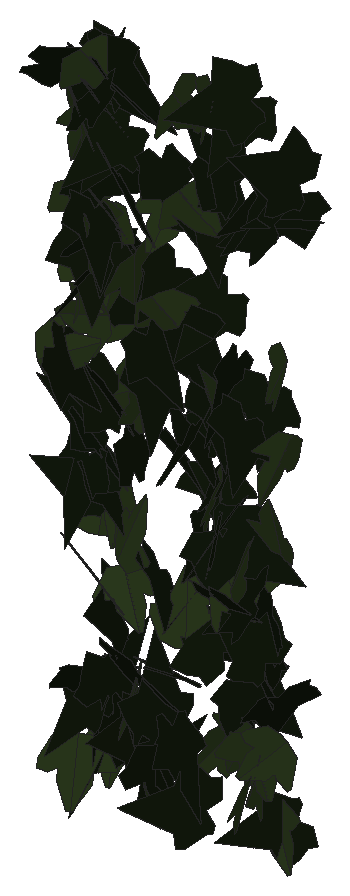
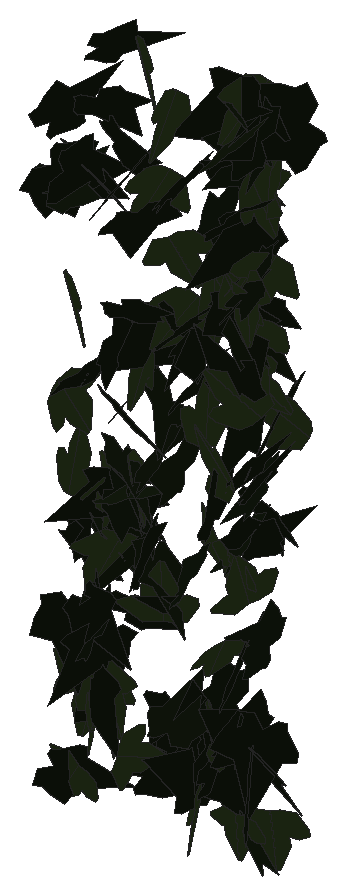
# SketchUp Ruby script. Lengths in inches.
U = 1.inch
M = Sketchup.active_model
def pt(a) = Geom::Point3d.new(a.map { |v| v * U })
def face(e, loops, mat)
  f = e.add_face(loops[0].map { |a| pt(a) })
  loops[1..].each { |l| e.add_face(l.map { |a| pt(a) }).erase! }
  f.material = f.back_material = mat if mat
  f
end
# faces: each face lists its corners as indices into pts; further lists are holes
def faces(e, pts, list, mat = nil) = list.each { |f| face(e, (f[0].is_a?(Array) ? f : [f]).map { |l| l.map { |i| pts[i] } }, mat) }
# xy, xz, yz: faces in a plane at the given z, y or x. An outline is a flat list of corners, or four numbers for a rectangle; further outlines are holes
def ring(l) = l.size == 4 ? [[l[0], l[1]], [l[2], l[1]], [l[2], l[3]], [l[0], l[3]]] : l.each_slice(2).to_a
def flat(e, list, mat, &to3) = list.each { |f| face(e, (f[0].is_a?(Array) ? f : [f]).map { |l| ring(l).map { |u, v| to3.(u, v) } }, mat) }
def xy(e, z, list, mat = nil) = flat(e, list, mat) { |x, y| [x, y, z] }
def xz(e, y, list, mat = nil) = flat(e, list, mat) { |x, z| [x, y, z] }
def yz(e, x, list, mat = nil) = flat(e, list, mat) { |y, z| [x, y, z] }
def lines(e, pts, list) = list.each { |a, b| e.add_line(pt(pts[a]), pt(pts[b])) }
# prism: a flat outline (further loops are holes) pulled along v
def prism(e, loops, v, mat = nil)
  f = face(e, loops, mat); d = Geom::Vector3d.new(v.map { |x| x * U })
  f.pushpull(f.normal.samedirection?(d) ? d.length : -d.length)
end
def box(e, o, s, mat = nil) = prism(e, [[o, [o[0] + s[0], o[1], o[2]], [o[0] + s[0], o[1] + s[1], o[2]], [o[0], o[1] + s[1], o[2]]]], [0, 0, s[2]], mat)
def at(x, y, z, deg = 0) = Geom::Transformation.translation(pt([x, y, z])) * Geom::Transformation.rotation(ORIGIN, Z_AXIS, deg.degrees)
def axes(o, x, y, z) = Geom::Transformation.new([*x, 0, *y, 0, *z, 0, *pt(o).to_a, 1])
def part(name) = M.definitions.add(name)
# library, detail: a bought-in or finely detailed component or shape, given as its bounding box
def library(name, o, s) = part(name).tap { |d| box(d.entities, o, s) }
def detail(e, o, s) = box(e.add_group.entities, o, s)
def put(e, d, t, mat = nil) = e.add_instance(d, t).tap { |i| i.material = mat if mat }
def group(e, t, mat = nil) = e.add_group.tap { |g| g.transformation = t; g.material = mat if mat }.entities
root = M.entities
M.materials.add("efeu1").color = [18, 25, 13]
M.materials.add("efeu2").color = [43, 57, 29]
c1 = part("ivyleaf_10")
p = [[0,0.5,-0.03],[-0.0625,2.02,-0.43],[-0.19,2.01,-0.46],[-0.54,1.05,-0.29],[-0.52,0.625,-0.18],[-0.83,0.76,-0.28],
  [-1.16,0.64,-0.33],[-1.15,0.33,-0.24],[-0.77,-0.39,0.02],[-0.3,-0.51,0.16],[0.04,-0.48,0.23],[-0.02,2.01,-0.4375],
  [-0.06,2.01,-0.43],[0.04,-0.49,0.23],[0.67,-0.49,0.14],[1.38,0.36,-0.2],[1.375,0.51,-0.24],[0.81,0.65,-0.19],
  [0.62,0.59,-0.15],[0.6,1.09,-0.28],[0.5,1.23,-0.31]]
faces(c1.entities,p,[[0,1,2,3,4,5,6,7,8,9,10],[11,12,0,13,14,15,16,17,18,19,20]],"efeu2")
c2 = part("ivyleaf_9")
p = [[1.54,2.16,1.25],[1.36,2.04,1.19],[-0.21,0.99,0.68],[-0.71,1.11,0.82],[-0.85,0.86,0.67],[-0.8,0.17,0.21],
  [-0.9,-0.01,0.1],[-0.67,-0.16,-0.02],[-0.08,-0.08,-0.05],[-0.03,-0.6,-0.4],[0.65,-0.88,-0.66],[0.83,-0.6,-0.49],
  [1.29,-0.42,-0.43],[1.8125,-0.07,-0.26],[1.21,0.44,0.15]]
faces(c2.entities,p,[[0,1,2,3,4,5,6,7,8,9,10,11,12,13,14]],"efeu1")
put(root,c1,axes([584.58,125.34,243.96],[1.0955,0.54995,-0.00416],[-0.00399,-0.00134,-1.22579],[-0.54995,1.0955,0.00059]))
put(root,c1,axes([583.95,124.68,261.51],[0.54254,-0.06384,-1.07288],[1.0655,-0.1256,0.54628],[-0.14089,-1.19567,-0.0001]))
put(root,c2,axes([584.14,123.93,274.76],[1.02793,0.37138,0.65667],[0.58931,0.29764,-1.09083],[-0.47101,1.18291,0.06831]))
put(root,c1,axes([584.64,125.48,268.77],[-0.86196,-0.52468,-0.46844],[0.52456,0.01409,-0.98099],[0.46858,-0.98093,0.23648]))
put(root,c1,axes([585.66,125.26,263.58],[0.41861,-0.1033,-1.10017],[-1.02006,0.41622,-0.42721],[0.42487,1.10107,0.05828]))
put(root,c1,axes([585.06,125.76,272.39],[-0.07314,-1.11185,0.34435],[-0.01366,-0.34419,-1.11422],[1.16387,-0.07391,0.00856]))
put(root,c2,axes([585.3,125.53,246.625],[-1.08694,0.11287,-0.22951],[0.22673,-0.03848,-1.09269],[-0.11836,-1.11024,0.01454]))
put(root,c2,axes([584.98,126.36,243.74],[-0.72617,0.2,-0.69404],[0.61757,-0.33844,-0.74369],[-0.37456,-0.94576,0.11936]))
put(root,c2,axes([585.09,125.35,247.72],[0.49911,1.03868,-0.22985],[-0.10203,-0.20597,-1.15237],[-1.0589,0.50943,0.0027]))
put(root,c1,axes([585.41,124.93,271.6],[-0.89919,0.64453,-0.4114],[-0.35391,0.21212,1.10588],[0.6778,0.96582,0.03166]))
put(root,c1,axes([585.42,126.1,267.99],[-1.08113,0.1071,0.42641],[-0.42702,0.01361,-1.08609],[-0.10464,-1.1621,0.02658]))
put(root,c2,axes([584.83,123.89,262.34],[0.77046,-0.53644,-0.92719],[-0.66912,0.65087,-0.93258],[0.8365,1.01472,0.10802]))
put(root,c2,axes([585.3,125.77,258.66],[0.06373,-1.18239,-0.08417],[0.03565,-0.08234,1.1837],[-1.18484,-0.06607,0.03109]))
put(root,c2,axes([584.4,127.07,246],[0.03478,-0.20714,-1.31804],[1.22225,-0.52375,0.11456],[-0.535,-1.21001,0.17604]))
put(root,c2,axes([585.39,126.4,259.47],[0.06632,-1.12656,-0.3189],[0.01473,-0.31859,1.12851],[-1.17074,-0.06783,-0.00387]))
put(root,c2,axes([584.37,125.91,252.13],[0.64336,-0.67956,0.58735],[0.42585,-0.40534,-0.93543],[0.79084,0.77109,0.0259]))
put(root,c2,axes([585.85,125.28,255.84],[-0.21206,0.21732,1.04453],[-0.99984,-0.41209,-0.11725],[0.37228,-0.98295,0.28009]))
put(root,c1,axes([585.23,126.02,254.13],[0.48224,0.98953,-0.45958],[0.1745,0.42605,1.10044],[1.07701,-0.5121,0.02749]))
put(root,c2,axes([584.62,126.13,268.57],[0.92581,-0.63304,0.22891],[0.17491,-0.14967,-1.12128],[0.65004,0.94187,-0.02432]))
put(root,c2,axes([585.81,125.49,265.9375],[-0.62118,0.66692,-0.67679],[0.23689,-0.67436,-0.88194],[-0.92017,-0.62383,0.22984]))
put(root,c1,axes([585.11,126.15,262.66],[-0.5218,-0.69168,0.777],[0.42472,0.65186,0.86551],[-0.94961,0.67162,-0.03984]))
put(root,c2,axes([585.77,125.53,266.82],[0.29725,0.91516,-0.57383],[-0.1381,-0.55808,-0.96158],[-1.07132,0.32586,-0.03526]))
put(root,c1,axes([585.27,126.62,244.25],[0.98544,0.08386,0.16592],[0.1662,0.00359,-0.98894],[-0.0833,0.9993,-0.01037]))
put(root,c1,axes([585.04,125.52,266.05],[1.02884,0.35447,0.46656],[0.44326,0.14572,-1.08817],[-0.3832,1.12024,-0.00608]))
put(root,c2,axes([585.6,126.875,271.09],[-0.49895,-0.93329,0.44428],[-0.03147,-0.47939,-1.04238],[1.03316,-0.46532,0.18281]))
put(root,c2,axes([585.14,125.18,258.84],[0.83061,-0.71632,-0.10791],[-0.06554,0.08919,-1.09655],[0.72143,0.83283,0.02462]))
put(root,c2,axes([585.4375,125.21,270.12],[0.10842,-0.01626,-1.24294],[-0.20746,1.22992,-0.03418],[1.22561,0.20963,0.10417]))
put(root,c2,axes([585.52,125.36,266.95],[-0.75343,-0.65875,-0.64537],[0.51421,0.3917,-1.00013],[0.76553,-0.91144,0.03663]))
put(root,c2,axes([585.6875,124.71,257.44],[-0.97025,-0.20215,-0.69409],[0.69891,0.03471,-0.98709],[0.18483,-1.19245,0.08893]))
put(root,c1,axes([585.7,125.13,266.61],[-0.75059,0.77432,0.53057],[0.37563,-0.3748,1.07837],[0.86022,0.83929,-0.00793]))
put(root,c2,axes([585.34,127.11,274.46],[-0.09012,-1.03828,0.50429],[0.28641,-0.51012,-0.9991],[1.11817,0.04699,0.29655]))
put(root,c2,axes([585.32,126.47,263.51],[-0.38171,0.23002,0.98589],[0.85188,-0.49631,0.44562],[0.54699,0.93347,-0.00601]))
put(root,c2,axes([585.44,125.85,267.45],[0.10794,-1.10129,0.33816],[0.07322,-0.33239,-1.10589],[1.14971,0.12456,0.03869]))
put(root,c2,axes([585.87,126.45,249.92],[-0.21225,-0.19899,1.26782],[-0.17045,-1.26929,-0.22776],[1.27197,-0.2033,0.18104]))
put(root,c2,axes([585.43,125.25,273.52],[1.01366,-0.56525,0.11525],[0.09838,-0.06021,-1.1606],[0.56843,1.01841,-0.00465]))
put(root,c1,axes([585.8125,126.04,267.57],[1.15166,-0.29752,0.30534],[0.29835,-0.06583,-1.18943],[0.30453,1.18963,0.01055]))
put(root,c1,axes([585.88,126.24,255.55],[1.04655,-0.28369,0.29762],[0.282,-0.09707,-1.08415],[0.29922,1.08371,-0.0192]))
put(root,c2,axes([585.74,125.08,268.29],[0.17254,-1.10914,0.18831],[0.05838,-0.18143,-1.1221],[1.1235,0.17976,0.02939]))
put(root,c2,axes([585.59,125.5,256.41],[0.73296,-0.91643,-0.02889],[-0.00582,0.03233,-1.17338],[0.91686,0.73282,0.01565]))
put(root,c2,axes([586.0625,125.16,246.96],[-0.22813,-0.20592,1.16272],[0.7954,0.84846,0.30633],[-0.87274,0.8271,-0.02475]))
put(root,c2,axes([585.26,125.34,274.24],[0.8398,-0.54203,0.77215],[0.66426,-0.39434,-0.99927],[0.66991,1.07051,0.02287]))
put(root,c2,axes([586.43,123.84,273.43],[-0.80658,0.92435,-0.04216],[-0.04474,0.01691,1.22657],[0.92423,0.8075,0.02259]))
put(root,c1,axes([586.08,124.32,275.6],[-0.72093,-0.6999,-0.70225],[0.55355,0.4362,-1.00302],[0.82255,-0.90699,0.05951]))
put(root,c2,axes([586.18,124.67,261.24],[1.01676,-0.10897,-0.45294],[-0.44897,0.06099,-1.02251],[0.12433,1.11141,0.01171]))
put(root,c1,axes([586.15,126.53,251.57],[-0.49536,-0.93083,0.02913],[0.67885,-0.3835,-0.71047],[0.63753,-0.3149,0.77914]))
put(root,c1,axes([585.76,126.91,259.51],[0.53955,-0.37826,-1.03324],[0.8582,-0.57551,0.65883],[-0.68859,-1.01365,0.01152]))
put(root,c2,axes([587.13,125.1875,272.43],[-1.07015,-0.40288,0.14132],[-0.13516,-0.04209,-1.14345],[0.40499,-1.07862,-0.00817]))
put(root,c2,axes([586.98,125.96,257.02],[-0.08991,-0.69281,0.9551],[0.26689,0.9211,0.69327],[-1.14933,0.26808,0.08627]))
put(root,c2,axes([585.89,124.8125,275.28],[0.00195,-0.10017,-1.50811],[1.15025,0.97844,-0.0635],[0.9805,-1.14764,0.07749]))
put(root,c2,axes([587.26,126.03,245.16],[-0.2373,-0.26128,1.03907],[-0.49205,-0.91881,-0.34341],[0.95175,-0.54017,0.08153]))
put(root,c2,axes([586.33,125.65,245.78],[-0.04623,-0.02844,-1.36092],[1.26623,0.49887,-0.05344],[0.49959,-1.26703,0.0095]))
put(root,c1,axes([587.15,125.27,246.26],[0.60095,-0.99484,0.15197],[-0.07297,0.13346,1.16224],[-1.00373,-0.60533,0.00649]))
put(root,c2,axes([586.47,125.45,248.5625],[0.99254,-0.45375,0.50394],[0.46914,-0.18557,-1.09108],[0.48965,1.09757,0.02386]))
put(root,c1,axes([587.5,125.23,266.58],[-0.01926,-1.1135,-0.2779],[0.03635,0.27721,-1.11324],[1.14707,-0.02748,0.03061]))
put(root,c2,axes([587.84,125.1875,268.83],[0.5622,-1.00976,0.55],[-0.24983,0.49033,1.15558],[-1.12237,-0.61494,0.01828]))
put(root,c1,axes([587.81,125.53,260.42],[-0.08517,-1.0748,-0.46005],[-0.05051,-0.45746,1.07809],[-1.16803,0.09816,-0.01307]))
put(root,c2,axes([587.85,127.31,265.54],[-0.37891,-0.87306,0.58255],[-0.00675,-0.61731,-0.92954],[1.04955,-0.31916,0.20434]))
put(root,c1,axes([588.47,125.11,243.59],[-0.57504,0.59245,0.81807],[-0.56591,0.59075,-0.82562],[-0.83664,-0.80679,-0.00381]))
put(root,c1,axes([587.69,124.59,254.31],[1.0104,-0.60019,-0.2963],[0.28471,-0.10019,1.17382],[-0.60578,-1.04818,0.05746]))
put(root,c2,axes([588.13,127.29,247.625],[-0.79722,-0.45824,0.46021],[0.45175,-0.91477,-0.12828],[0.46658,0.10273,0.91055]))
put(root,c1,axes([588.375,126.625,269.02],[0.86834,0.59442,-0.39867],[-0.35177,-0.19144,-1.05161],[-0.62332,0.93611,0.03809]))
put(root,c2,axes([588.68,125.51,246.46],[-0.55177,-0.80181,0.80469],[0.45735,0.66209,0.97332],[-1.03984,0.71667,0.00109]))
put(root,c2,axes([588.46,124.6875,244.2],[0.04093,-0.01153,1.22765],[0.84868,0.88784,-0.01996],[-0.88712,0.84884,0.03755]))
put(root,c2,axes([588.28,126.34,258.75],[0.65465,-0.75717,0.41916],[0.29682,-0.29726,-1.00055],[0.81296,0.71826,0.02777]))
put(root,c2,axes([588.66,125.09,262.08],[0.13337,-1.12104,0.29146],[-0.00583,-0.29403,-1.12827],[1.1583,0.1276,-0.03923]))
put(root,c2,axes([588.9,124.42,264.03],[0.37695,-0.84749,-0.6327],[-0.23595,0.58737,-0.92735],[1.03096,0.4443,0.0191]))
put(root,c2,axes([588.82,125.45,271.35],[0.46319,-1.02496,-0.33515],[-0.06785,0.33633,-1.12236],[1.07623,0.46233,0.07348]))
put(root,c1,axes([589.03,125.05,265.31],[-0.87708,-0.36223,-0.60321],[0.5578,0.22962,-0.94894],[0.42888,-1.03943,0.00058]))
put(root,c2,axes([588.74,125.33,253.32],[0.26192,-0.88321,0.69389],[0.18385,-0.66918,-0.92116],[1.10803,0.31982,-0.01118]))
put(root,c1,axes([589.43,125.49,274.4],[-0.03517,-0.94096,-0.68531],[0.22205,0.66761,-0.92805],[1.14269,-0.15869,0.15925]))
put(root,c2,axes([589.02,126.72,259.39],[0.65913,-0.92377,0.09274],[0.0575,-0.0729,-1.1348],[0.92663,0.66162,0.00445]))
put(root,c2,axes([589.4,125.45,264.4],[-0.2322,-0.39322,-1.34017],[0.96815,0.93388,-0.44176],[1.00666,-0.98886,0.11573]))
put(root,c2,axes([589.65,125.09,246.66],[-0.51905,-0.1734,-1.15273],[1.08638,0.38553,-0.54717],[0.42263,-1.20397,-0.00919]))
put(root,c2,axes([589.87,126.86,254.64],[0.28746,-0.43677,-1.01931],[0.81489,-0.63099,0.50019],[-0.75214,-0.85057,0.15235]))
put(root,c1,axes([590.24,125.11,251.28],[1.07847,0.66947,-0.05661],[0.0408,0.04161,1.26929],[0.67062,-1.07915,0.01383]))
put(root,c1,axes([590.53,127.0625,245.58],[0.03537,0.44837,-0.96186],[-0.39352,-0.88824,-0.42852],[-0.98557,0.37075,0.13658]))
put(root,c2,axes([591.04,125.12,243.625],[-0.41415,-0.24688,1.06482],[-0.95605,-0.47018,-0.48085],[0.52988,-1.0413,-0.03533]))
put(root,c2,axes([590.97,124.62,253.3],[-0.53942,1.07353,-0.03794],[0.00984,-0.03752,-1.20141],[-1.07416,-0.53945,0.00805]))
put(root,c2,axes([590.9375,123.69,259.76],[-0.01283,0.91777,0.91135],[-0.13182,0.90572,-0.91396],[-1.28666,-0.10195,0.08455]))
put(root,c2,axes([590.75,126.83,265.5],[-0.95648,-0.53684,0.00004],[0.07213,-0.12859,-1.08688],[0.53197,-0.94779,0.14744]))
put(root,c1,axes([590.31,125.08,270.46],[-0.59663,-0.74729,-0.61186],[0.51563,0.36167,-0.94451],[0.81666,-0.77429,0.14934]))
put(root,c2,axes([590.3,126.59,269.6875],[-0.23616,-1.04544,-0.38737],[0.10742,0.37278,-1.07158],[1.10972,-0.25857,0.02129]))
put(root,c2,axes([591.62,126.28,260.42],[-0.67189,0.58417,0.59683],[-0.49211,0.34196,-0.8887],[-0.67475,-0.83109,0.05385]))
put(root,c2,axes([590.3125,127.11,257.24],[-0.24367,-1.0315,0.11494],[0.57234,-0.23203,-0.869],[0.86581,-0.13691,0.6068]))
put(root,c2,axes([591.53,125.92,258.18],[-0.51332,0.96456,0.35543],[-0.2209,0.28449,-1.09109],[-1.00395,-0.55578,0.05835]))
put(root,c2,axes([591.71,125.36,250.82],[-0.9304,-0.51547,-0.35197],[-0.30825,-0.16989,1.06365],[-0.54274,0.98014,-0.00074]))
put(root,c1,axes([591,125.43,262.5],[-0.9992,0.52266,0.0024],[-0.00216,0.00105,-1.12764],[-0.52266,-0.99921,0.00007]))
put(root,c1,axes([591.16,125.78,257.57],[0.49501,-0.99677,-0.19402],[-0.10269,0.1656,-1.11277],[1.01027,0.50522,-0.01804]))
put(root,c2,axes([590.7,126.15,261.48],[0.30906,-1.08031,0.19513],[0.07141,-0.1825,-1.12351],[1.09547,0.31668,0.01819]))
put(root,c2,axes([592.21,125.5,271.76],[-0.88277,0.04613,-0.82764],[-0.82626,-0.14579,0.87318],[-0.06638,1.20126,0.13776]))
put(root,c2,axes([590.79,126.125,271.46],[0.68407,-0.93214,-0.41267],[-0.1342,0.41031,-1.14925],[1.01054,0.68549,0.12674]))
put(root,c1,axes([591.77,124.47,275.58],[0.64815,-0.75709,-0.57442],[-0.35203,0.45457,-0.99634],[0.88274,0.73717,0.02444]))
put(root,c2,axes([591.74,126.16,256.55],[-0.70857,0.42285,-0.78669],[0.48242,-0.66391,-0.79137],[-0.75164,-0.82473,0.23371]))
put(root,c2,axes([592.02,124.38,255.49],[0.11069,0.069,1.1975],[-0.07902,1.20039,-0.06186],[-1.19688,-0.07287,0.11483]))
put(root,c2,axes([591.91,126.97,274.49],[-0.86635,-0.7284,-0.03226],[0.02725,0.01771,-1.13186],[0.72861,-0.86676,0.00398]))
put(root,c2,axes([592.04,125.93,263.34],[-0.16698,0.2072,-1.16645],[0.82804,-0.82206,-0.26456],[-0.84729,-0.84422,-0.02867]))
put(root,c2,axes([593.07,126.34,251.1875],[0.06508,0.22115,-1.08745],[-0.99478,-0.47113,-0.15535],[-0.49179,0.98225,0.17033]))
put(root,c1,axes([592.97,125.57,247.44],[-1.00764,-0.19474,0.58965],[-0.57119,-0.15027,-1.02572],[0.24362,-1.15777,0.03396]))
put(root,c2,axes([593.1,125.29,275.66],[-0.73246,-0.31815,0.86652],[-0.65274,-0.60363,-0.77339],[0.65269,-0.96072,0.19897]))
put(root,c2,axes([592.28,124.25,254.01],[1.23542,0.24901,-0.29936],[-0.33473,0.17039,-1.23968],[-0.19893,1.2597,0.22686]))
put(root,c2,axes([593.21,125.72,247.26],[0.32476,0.26357,-1.06223],[-1.03324,-0.29149,-0.38822],[-0.36085,1.07183,0.15563]))
put(root,c2,axes([591.89,125.05,256.2],[0.32779,-0.4149,-1.23904],[0.49595,1.22135,-0.27777],[1.20889,-0.38856,0.44992]))
put(root,c1,axes([592.44,125.36,253.625],[0.49973,0.9962,0.5115],[0.19977,0.47184,-1.11411],[-1.10188,0.53734,0.03]))
put(root,c2,axes([592.71,125.73,249.57],[0.0985,-0.50179,-1.10592],[-0.16437,1.09383,-0.51094],[1.20326,0.19049,0.02073]))
put(root,c2,axes([593.27,127.33,270.875],[-0.1954,-0.28508,-1.11096],[0.40261,-1.0723,0.20435],[-1.07397,-0.35011,0.27874]))
put(root,c2,axes([593.87,124.65,254.08],[-0.92747,0.73043,0.11664],[-0.09032,0.07384,-1.18057],[-0.73415,-0.93186,-0.00212]))
put(root,c2,axes([592.88,126.98,261.86],[-0.18863,-1.08534,0.18352],[0.07752,-0.19883,-1.09621],[1.09802,-0.17242,0.10892]))
put(root,c2,axes([592.55,126.56,250.01],[0.27279,-0.67801,0.87201],[0.37811,-0.78663,-0.72991],[1.03785,0.4648,0.03672]))
put(root,c1,axes([593.6,124.14,255.13],[0.31445,-0.24174,1.10037],[-0.65197,0.89265,0.38242],[-0.9188,-0.71615,0.10523]))
put(root,c2,axes([594.21,125.45,270.49],[-0.90273,0.64888,0.27047],[-0.26304,0.09646,-1.10934],[-0.65193,-0.93743,0.07306]))
put(root,c1,axes([593.49,125.27,247.29],[-1.16284,-0.47732,-0.17273],[0.20073,-0.03584,-1.25231],[0.46623,-1.17505,0.10836]))
put(root,c1,axes([593.61,124.54,245.78],[0.44597,-1.02818,-0.13222],[-0.04558,0.12435,-1.12071],[1.03564,0.44823,0.00761]))
put(root,c2,axes([593.18,125.04,261.53],[-0.01661,-1.06986,0.41077],[0.02109,-0.41103,-1.06968],[1.14581,-0.00794,0.02565]))
put(root,c2,axes([593.91,127.29,270.86],[-0.01979,0.05104,-1.25533],[0.01016,-1.25544,-0.05121],[-1.25633,-0.01095,0.01936]))
put(root,c1,axes([593.2,125.96,245.52],[0.00325,0.02338,-1.17165],[0.29036,-1.13513,-0.02185],[-1.13534,-0.29024,-0.00894]))
put(root,c2,axes([594.28,126.6875,243.57],[-0.14341,-0.27349,-1.03819],[-0.41922,-0.94999,0.30817],[-0.98838,0.44262,0.01993]))
put(root,c2,axes([593.93,127.46,269.83],[-0.99999,-0.44485,0.18199],[0.37454,-0.98451,-0.3485],[0.30121,-0.25267,1.03751]))
put(root,c2,axes([594.7,124.26,251.94],[-0.21449,0.37712,1.0581],[-0.95801,0.50106,-0.37278],[-0.58654,-0.95631,0.22194]))
put(root,c1,axes([594.16,125.8,256.14],[-1.11757,0.22641,0.0382],[0.03326,-0.0282,1.14008],[0.22719,1.11787,0.02102]))
put(root,c1,axes([593.46,126.44,243.5625],[0.89974,0.00361,0.67761],[0.67753,-0.02266,-0.89952],[0.01075,1.12613,-0.02028]))
put(root,c2,axes([594.74,124.74,253.65],[0.10793,0.09878,-1.11888],[-1.12311,-0.00721,-0.10897],[-0.01669,1.12405,0.09763]))
put(root,c1,axes([594.16,126.27,260.25],[-0.11228,-1.01517,0.57829],[0.08775,-0.58665,-1.01279],[1.16503,-0.05365,0.13201]))
put(root,c1,axes([594.78,124.96,247.6875],[0.86422,-0.01464,-0.74475],[-0.74094,0.10058,-0.86177],[0.07671,1.13641,0.06668]))
put(root,c2,axes([594.81,126.23,272.23],[-0.21021,0.0878,1.18135],[-0.8925,-0.80066,-0.0993],[0.77893,-0.89371,0.20502]))
put(root,c1,axes([594.68,125.33,264.38],[0.6796,-0.81501,-0.49024],[-0.30653,0.3827,-1.06114],[0.90034,0.74548,0.00878]))
put(root,c2,axes([594.73,125.21,249.8],[0.13237,1.08542,-0.29619],[-0.03441,-0.29419,-1.09346],[-1.12458,0.13676,-0.0014]))
